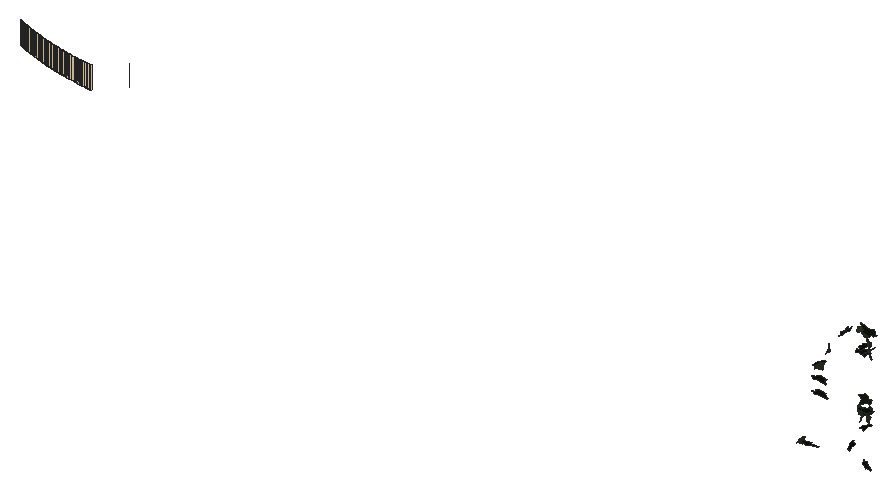
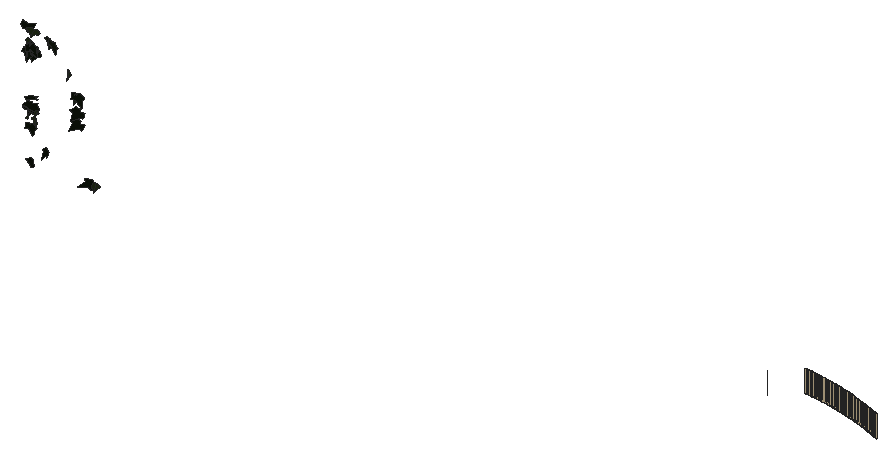
# SketchUp Ruby script. Lengths in inches.
U = 1.inch
M = Sketchup.active_model
def pt(a) = Geom::Point3d.new(a.map { |v| v * U })
def face(e, loops, mat)
  f = e.add_face(loops[0].map { |a| pt(a) })
  loops[1..].each { |l| e.add_face(l.map { |a| pt(a) }).erase! }
  f.material = f.back_material = mat if mat
  f
end
# faces: each face lists its corners as indices into pts; further lists are holes
def faces(e, pts, list, mat = nil) = list.each { |f| face(e, (f[0].is_a?(Array) ? f : [f]).map { |l| l.map { |i| pts[i] } }, mat) }
# xy, xz, yz: faces in a plane at the given z, y or x. An outline is a flat list of corners, or four numbers for a rectangle; further outlines are holes
def ring(l) = l.size == 4 ? [[l[0], l[1]], [l[2], l[1]], [l[2], l[3]], [l[0], l[3]]] : l.each_slice(2).to_a
def flat(e, list, mat, &to3) = list.each { |f| face(e, (f[0].is_a?(Array) ? f : [f]).map { |l| ring(l).map { |u, v| to3.(u, v) } }, mat) }
def xy(e, z, list, mat = nil) = flat(e, list, mat) { |x, y| [x, y, z] }
def xz(e, y, list, mat = nil) = flat(e, list, mat) { |x, z| [x, y, z] }
def yz(e, x, list, mat = nil) = flat(e, list, mat) { |y, z| [x, y, z] }
def lines(e, pts, list) = list.each { |a, b| e.add_line(pt(pts[a]), pt(pts[b])) }
# prism: a flat outline (further loops are holes) pulled along v
def prism(e, loops, v, mat = nil)
  f = face(e, loops, mat); d = Geom::Vector3d.new(v.map { |x| x * U })
  f.pushpull(f.normal.samedirection?(d) ? d.length : -d.length)
end
def box(e, o, s, mat = nil) = prism(e, [[o, [o[0] + s[0], o[1], o[2]], [o[0] + s[0], o[1] + s[1], o[2]], [o[0], o[1] + s[1], o[2]]]], [0, 0, s[2]], mat)
def at(x, y, z, deg = 0) = Geom::Transformation.translation(pt([x, y, z])) * Geom::Transformation.rotation(ORIGIN, Z_AXIS, deg.degrees)
def axes(o, x, y, z) = Geom::Transformation.new([*x, 0, *y, 0, *z, 0, *pt(o).to_a, 1])
def part(name) = M.definitions.add(name)
# library, detail: a bought-in or finely detailed component or shape, given as its bounding box
def library(name, o, s) = part(name).tap { |d| box(d.entities, o, s) }
def detail(e, o, s) = box(e.add_group.entities, o, s)
def put(e, d, t, mat = nil) = e.add_instance(d, t).tap { |i| i.material = mat if mat }
def group(e, t, mat = nil) = e.add_group.tap { |g| g.transformation = t; g.material = mat if mat }.entities
root = M.entities
M.materials.add("1026 AP 7946 SUNNY SIDE UP").color = [254, 231, 186]
M.materials.add("efeu1").color = [18, 25, 13]
M.materials.add("efeu2").color = [43, 57, 29]
c1 = part("ivyleaf_10")
p = [[0,0.5,-0.03],[-0.0625,2.02,-0.43],[-0.19,2.01,-0.46],[-0.54,1.05,-0.29],[-0.52,0.625,-0.18],[-0.83,0.76,-0.28],
  [-1.16,0.64,-0.33],[-1.15,0.33,-0.24],[-0.77,-0.39,0.02],[-0.3,-0.51,0.16],[0.04,-0.48,0.23],[-0.02,2.01,-0.4375],
  [-0.06,2.01,-0.43],[0.04,-0.49,0.23],[0.67,-0.49,0.14],[1.38,0.36,-0.2],[1.375,0.51,-0.24],[0.81,0.65,-0.19],
  [0.62,0.59,-0.15],[0.6,1.09,-0.28],[0.5,1.23,-0.31]]
faces(c1.entities,p,[[0,1,2,3,4,5,6,7,8,9,10],[11,12,0,13,14,15,16,17,18,19,20]],"efeu2")
c2 = part("ivyleaf_9")
p = [[1.54,2.16,1.25],[1.36,2.04,1.19],[-0.21,0.99,0.68],[-0.71,1.11,0.82],[-0.85,0.86,0.67],[-0.8,0.17,0.21],
  [-0.9,-0.01,0.1],[-0.67,-0.16,-0.02],[-0.08,-0.08,-0.05],[-0.03,-0.6,-0.4],[0.65,-0.88,-0.66],[0.83,-0.6,-0.49],
  [1.29,-0.42,-0.43],[1.8125,-0.07,-0.26],[1.21,0.44,0.15]]
faces(c2.entities,p,[[0,1,2,3,4,5,6,7,8,9,10,11,12,13,14]],"efeu1")
p = [[27.242,213.147,276],[27.198,213.151,276],[27.198,213.151,274],[27.242,213.147,274],[27.282,213.142,276],[27.282,213.142,274],
  [27.36,213.135,276],[27.36,213.135,274],[27.452,213.125,276],[27.452,213.125,274],[27.505,213.12,276],[27.505,213.12,274],
  [27.553,213.115,276],[27.553,213.115,274],[27.624,213.109,276],[27.624,213.109,274],[27.706,213.101,276],[27.706,213.101,274],
  [27.768,213.096,276],[27.768,213.096,274],[27.824,213.091,276],[27.824,213.091,274],[27.888,213.086,276],[27.888,213.086,274],
  [26.4375,213.245,276],[26.284,213.267,276],[26.284,213.267,274],[26.4375,213.245,274],[26.455,213.243,276],[26.455,213.243,274],
  [26.471,213.241,276],[26.471,213.241,274],[26.561,213.229,276],[26.561,213.229,274],[26.691,213.211,276],[26.691,213.211,274],
  [26.717,213.208,276],[26.717,213.208,274],[26.741,213.205,276],[26.741,213.205,274],[26.83,213.194,276],[26.83,213.194,274],
  [26.944,213.18,276],[26.944,213.18,274],[26.979,213.176,276],[26.979,213.176,274],[27.012,213.172,276],[27.012,213.172,274],
  [27.095,213.163,276],[27.095,213.163,274],[25.933,213.32,276],[25.681,213.361,276],[25.681,213.361,274],[25.933,213.32,274],
  [26.185,213.281,276],[26.185,213.281,274],[26.193,213.28,276],[26.193,213.28,274],[26.202,213.279,276],[26.202,213.279,274],
  [25.307,213.427,276],[25.178,213.451,276],[25.178,213.451,274],[25.307,213.427,274],[25.396,213.411,276],[25.396,213.411,274],
  [25.412,213.408,276],[25.412,213.408,274],[25.429,213.405,276],[25.429,213.405,274],[25.582,213.378,276],[25.582,213.378,274],
  [25.664,213.364,276],[25.664,213.364,274],[25.672,213.363,276],[25.672,213.363,274],[24.778,213.53,276],[24.678,213.551,276],
  [24.678,213.551,274],[24.778,213.53,274],[24.861,213.513,276],[24.861,213.513,274],[24.893,213.507,276],[24.893,213.507,274],
  [24.928,213.5,276],[24.928,213.5,274],[25.041,213.478,276],[25.041,213.478,274],[25.128,213.461,276],[25.128,213.461,274],
  [25.153,213.456,276],[25.153,213.456,274],[24.259,213.642,276],[24.179,213.66,276],[24.179,213.66,274],[24.259,213.642,274],
  [24.328,213.626,276],[24.328,213.626,274],[24.376,213.616,276],[24.376,213.616,274],[24.428,213.604,276],[24.428,213.604,274],
  [24.518,213.585,276],[24.518,213.585,274],[24.594,213.568,276],[24.594,213.568,274],[24.634,213.56,276],[24.634,213.56,274],
  [23.861,213.735,276],[23.798,213.75,276],[23.798,213.75,274],[23.861,213.735,274],[23.93,213.718,276],[23.93,213.718,274],
  [24,213.702,276],[24,213.702,274],[24.063,213.687,276],[24.063,213.687,274],[24.118,213.674,276],[24.118,213.674,274],
  [23.435,213.842,276],[23.346,213.866,276],[23.346,213.866,274],[23.435,213.842,274],[23.487,213.829,276],[23.487,213.829,274],
  [23.534,213.817,276],[23.534,213.817,274],[23.603,213.799,276],[23.603,213.799,274],[23.683,213.779,276],[23.683,213.779,274],
  [23.743,213.764,276],[23.743,213.764,274],[23.089,213.935,276],[23.008,213.958,276],[23.008,213.958,274],[23.089,213.935,274],
  [23.189,213.908,276],[23.189,213.908,274],[23.231,213.897,276],[23.231,213.897,274],[23.271,213.886,276],[23.271,213.886,274],
  [22.697,214.047,276],[22.572,214.084,276],[22.572,214.084,274],[22.697,214.047,274],[22.722,214.039,276],[22.722,214.039,274],
  [22.746,214.032,276],[22.746,214.032,274],[22.832,214.008,276],[22.832,214.008,274],[22.943,213.976,276],[22.943,213.976,274],
  [22.976,213.967,276],[22.976,213.967,274],[22.453,214.12,276],[22.304,214.165,276],[22.304,214.165,274],[22.453,214.12,274],
  [22.469,214.115,276],[22.469,214.115,274],[22.485,214.11,276],[22.485,214.11,274],[22.209,214.195,276],[21.966,214.273,276],
  [21.966,214.273,274],[22.209,214.195,274],[22.217,214.192,276],[22.217,214.192,274],[22.225,214.19,276],[22.225,214.19,274],
  [21.723,214.353,276],[21.723,214.353,274],[21.449,214.446,276],[21.364,214.476,276],[21.364,214.476,274],[21.449,214.446,274],
  [21.465,214.441,276],[21.465,214.441,274],[21.482,214.435,276],[21.482,214.435,274],[21.629,214.385,276],[21.629,214.385,274],
  [21.707,214.358,276],[21.707,214.358,274],[21.715,214.355,276],[21.715,214.355,274],[21.193,214.537,276],[21.109,214.568,276],
  [21.109,214.568,274],[21.193,214.537,274],[21.216,214.529,276],[21.216,214.529,274],[21.241,214.52,276],[21.241,214.52,274],
  [20.937,214.631,276],[20.858,214.66,276],[20.858,214.66,274],[20.937,214.631,274],[20.968,214.619,276],[20.968,214.619,274],
  [21.001,214.607,276],[21.001,214.607,274],[20.682,214.727,276],[20.609,214.755,276],[20.609,214.755,274],[20.682,214.727,274],
  [20.721,214.712,276],[20.721,214.712,274],[20.762,214.697,276],[20.762,214.697,274],[20.429,214.826,276],[20.362,214.852,276],
  [20.362,214.852,274],[20.429,214.826,274],[20.474,214.808,276],[20.474,214.808,274],[20.524,214.788,276],[20.524,214.788,274],
  [20.176,214.927,276],[20.117,214.952,276],[20.117,214.952,274],[20.176,214.927,274],[20.229,214.906,276],[20.229,214.906,274],
  [20.287,214.883,276],[20.287,214.883,274],[19.925,215.032,276],[19.872,215.054,276],[19.872,215.054,274],[19.925,215.032,274],
  [19.984,215.007,276],[19.984,215.007,274],[20.05,214.979,276],[20.05,214.979,274],[29.764,215.001,274],[29.764,215.001,276]]
faces(root,p,[[0,1,2,3],[4,0,3,5],[6,4,5,7],[8,6,7,9],[10,8,9,11],[12,10,11,13],[14,12,13,15],[16,14,15,17],
  [18,16,17,19],[20,18,19,21],[22,20,21,23],[24,25,26,27],[28,24,27,29],[30,28,29,31],[32,30,31,33],[34,32,33,35],
  [36,34,35,37],[38,36,37,39],[40,38,39,41],[42,40,41,43],[44,42,43,45],[46,44,45,47],[48,46,47,49],[1,48,49,2],
  [50,51,52,53],[54,50,53,55],[56,54,55,57],[58,56,57,59],[25,58,59,26],[60,61,62,63],[64,60,63,65],[66,64,65,67],
  [68,66,67,69],[70,68,69,71],[72,70,71,73],[74,72,73,75],[51,74,75,52],[76,77,78,79],[80,76,79,81],[82,80,81,83],
  [84,82,83,85],[86,84,85,87],[88,86,87,89],[90,88,89,91],[61,90,91,62],[92,93,94,95],[96,92,95,97],[98,96,97,99],
  [100,98,99,101],[102,100,101,103],[104,102,103,105],[106,104,105,107],[77,106,107,78],[108,109,110,111],[112,108,111,113],[114,112,113,115],
  [116,114,115,117],[118,116,117,119],[93,118,119,94],[120,121,122,123],[124,120,123,125],[126,124,125,127],[128,126,127,129],[130,128,129,131],
  [132,130,131,133],[109,132,133,110],[134,135,136,137],[138,134,137,139],[140,138,139,141],[142,140,141,143],[121,142,143,122],[144,145,146,147],
  [148,144,147,149],[150,148,149,151],[152,150,151,153],[154,152,153,155],[156,154,155,157],[135,156,157,136],[158,159,160,161],[162,158,161,163],
  [164,162,163,165],[145,164,165,146],[166,167,168,169],[170,166,169,171],[172,170,171,173],[159,172,173,160],[167,174,175,168],[176,177,178,179],
  [180,176,179,181],[182,180,181,183],[184,182,183,185],[186,184,185,187],[188,186,187,189],[174,188,189,175],[190,191,192,193],[194,190,193,195],
  [196,194,195,197],[177,196,197,178],[198,199,200,201],[202,198,201,203],[204,202,203,205],[191,204,205,192],[206,207,208,209],[210,206,209,211],
  [212,210,211,213],[199,212,213,200],[214,215,216,217],[218,214,217,219],[220,218,219,221],[207,220,221,208],[222,223,224,225],[226,222,225,227],
  [228,226,227,229],[215,228,229,216],[230,231,232,233],[234,230,233,235],[236,234,235,237],[223,236,237,224]],"1026 AP 7946 SUNNY SIDE UP")
lines(root,p,[[238,239]])
put(root,c1,axes([92.16,213.08,268.27],[-0.08668,-0.23302,-0.09001],[0.06668,0.07802,-0.24519],[0.38485,-0.066,0.02221]),"1026 AP 7946 SUNNY SIDE UP")
put(root,c2,axes([92.53,213,268.16],[0.3572,0.01693,0.12122],[0.17822,0.04502,-0.23203],[-0.05589,0.2518,0.03486]),"1026 AP 7946 SUNNY SIDE UP")
put(root,c2,axes([93.71,213.15,275],[0.01581,0.27775,-0.06445],[-0.0469,-0.0628,-0.28535],[-0.44576,0.01646,0.02774]),"1026 AP 7946 SUNNY SIDE UP")
put(root,c2,axes([93.5,213.16,273.74],[0.40746,0.10638,-0.0076],[0.00457,-0.02798,-0.2874],[-0.16768,0.25774,-0.02629]),"1026 AP 7946 SUNNY SIDE UP")
put(root,c2,axes([93.62,212.99,272.67],[0.41378,0.08324,0.03384],[0.05663,-0.00671,-0.28382],[-0.12851,0.26505,-0.01611]),"1026 AP 7946 SUNNY SIDE UP")
put(root,c1,axes([93.81,213.11,274.9],[-0.14368,-0.24748,-0.11228],[0.09826,0.09109,-0.27001],[0.41278,-0.10783,0.02519]),"1026 AP 7946 SUNNY SIDE UP")
put(root,c1,axes([94.625,213.04,276.53],[0.07051,-0.23476,-0.17481],[0.0075,0.17095,-0.24327],[0.45419,0.03363,0.03116]),"1026 AP 7946 SUNNY SIDE UP")
put(root,c2,axes([96.08,212.99,278.35],[-0.06469,0.25385,0.10034],[-0.01404,0.09017,-0.2735],[-0.45722,-0.03869,-0.0058]),"1026 AP 7946 SUNNY SIDE UP")
put(root,c2,axes([96.25,212.98,278.43],[0.08951,0.2043,0.18645],[-0.0134,0.17593,-0.21933],[-0.45261,0.03519,0.04337]),"1026 AP 7946 SUNNY SIDE UP")
put(root,c2,axes([96.66,212.98,269.4],[-0.01521,0.04227,-0.26775],[-0.24234,0.21026,0.04233],[0.33616,0.15349,0.0184]),"1026 AP 7946 SUNNY SIDE UP")
put(root,c1,axes([97.48,213.22,271.74],[0.06224,0.11379,0.2113],[-0.23538,0.16819,-0.07446],[-0.3041,-0.10689,0.10089]),"1026 AP 7946 SUNNY SIDE UP")
put(root,c1,axes([97.32,213.17,272.46],[-0.03898,0.23426,0.0494],[-0.00051,0.04326,-0.25136],[-0.40434,-0.02264,-0.00444]),"1026 AP 7946 SUNNY SIDE UP")
put(root,c2,axes([97.51,213.2,277.26],[0.32238,0.15588,-0.06508],[-0.07218,-0.04715,-0.2635],[-0.27601,0.19439,-0.00711]),"1026 AP 7946 SUNNY SIDE UP")
put(root,c2,axes([97.71,213.39,277.74],[0.01103,0.22315,-0.13627],[-0.02069,-0.12983,-0.24068],[-0.43807,0.01175,0.00794]),"1026 AP 7946 SUNNY SIDE UP")
put(root,c1,axes([97.49,213.29,279.01],[0.38403,0.09135,0.10102],[0.12268,0.06755,-0.25782],[-0.18442,0.23516,0.03886]),"1026 AP 7946 SUNNY SIDE UP")
put(root,c2,axes([97.6875,213.02,277.56],[0.14752,0.19895,0.16043],[0.03484,0.14975,-0.22746],[-0.41874,0.08255,0.03759]),"1026 AP 7946 SUNNY SIDE UP")
put(root,c2,axes([97.82,213.29,271.22],[0.05409,0.2132,-0.06785],[-0.01174,-0.06585,-0.23168],[-0.37875,0.03249,-0.00251]),"1026 AP 7946 SUNNY SIDE UP")
put(root,c2,axes([98.07,213.28,272.375],[-0.09314,0.1144,0.20552],[-0.31179,0.08705,-0.1114],[-0.21224,-0.17809,0.07346]),"1026 AP 7946 SUNNY SIDE UP")
put(root,c2,axes([97.95,213.29,273.48],[-0.30431,-0.12979,0.0806],[-0.08098,-0.06466,-0.23655],[0.24302,-0.18407,0.0221]),"1026 AP 7946 SUNNY SIDE UP")
put(root,c2,axes([97.93,213.44,277.24],[0.09198,0.23517,0.08772],[0.02913,0.07698,-0.25729],[-0.42006,0.05684,0.00136]),"1026 AP 7946 SUNNY SIDE UP")
put(root,c2,axes([97.9,212.97,272.76],[0.32997,0.16855,-0.07706],[-0.10314,-0.03922,-0.27732],[-0.27165,0.21963,0.0117]),"1026 AP 7946 SUNNY SIDE UP")
put(root,c1,axes([97.92,213.37,278.08],[-0.27741,0.20052,-0.01199],[-0.025,-0.0297,-0.27547],[-0.34029,-0.16129,0.03001]),"1026 AP 7946 SUNNY SIDE UP")
put(root,c1,axes([98.07,213.38,277.12],[-0.20109,0.19064,0.13465],[-0.13007,0.09733,-0.23858],[-0.36278,-0.14057,0.01091]),"1026 AP 7946 SUNNY SIDE UP")
put(root,c2,axes([97.74,213.23,268.21],[0.09804,-0.03786,-0.21911],[0.35089,-0.00977,0.0644],[-0.03368,-0.21196,0.03311]),"1026 AP 7946 SUNNY SIDE UP")
put(root,c1,axes([98.03,213.22,272.08],[-0.0537,0.2224,-0.04202],[0.00078,-0.04249,-0.24101],[-0.38425,-0.03117,0.00539]),"1026 AP 7946 SUNNY SIDE UP")
put(root,c2,axes([98.31,213.15,278.9],[0.13945,-0.04369,0.27367],[-0.34754,0.15464,0.10067],[-0.27178,-0.22017,0.01169]),"1026 AP 7946 SUNNY SIDE UP")
